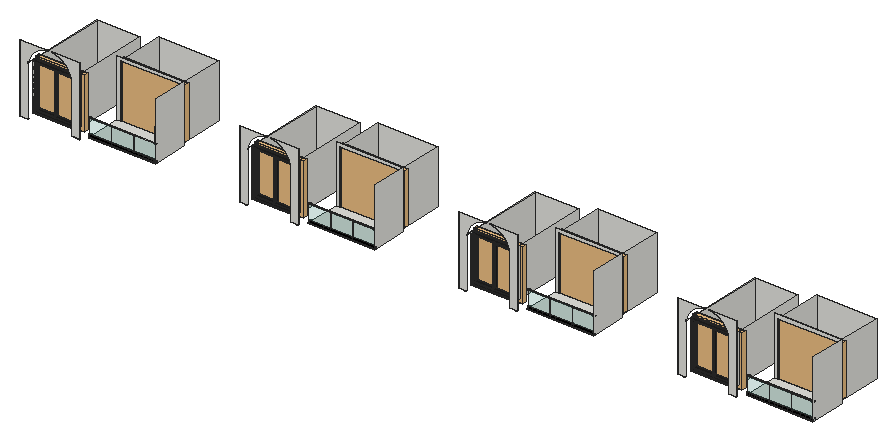
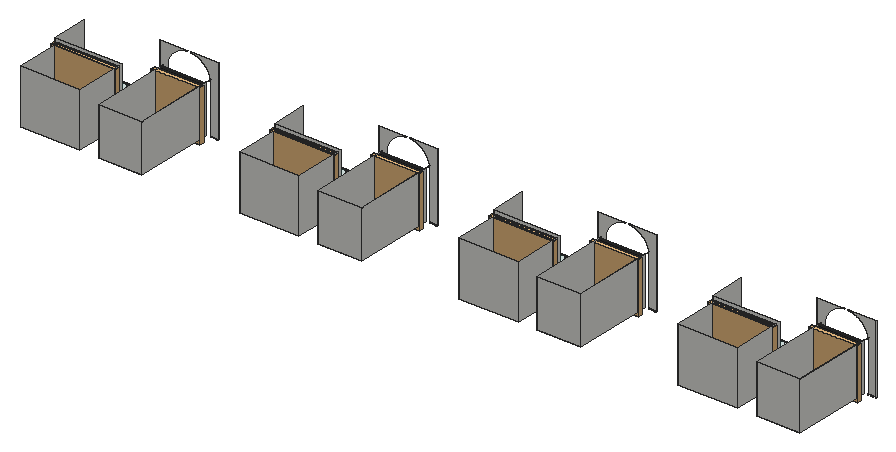
# SketchUp Ruby script. Lengths in inches.
U = 1.inch
M = Sketchup.active_model
def pt(a) = Geom::Point3d.new(a.map { |v| v * U })
def face(e, loops, mat)
  f = e.add_face(loops[0].map { |a| pt(a) })
  loops[1..].each { |l| e.add_face(l.map { |a| pt(a) }).erase! }
  f.material = f.back_material = mat if mat
  f
end
# faces: each face lists its corners as indices into pts; further lists are holes
def faces(e, pts, list, mat = nil) = list.each { |f| face(e, (f[0].is_a?(Array) ? f : [f]).map { |l| l.map { |i| pts[i] } }, mat) }
# xy, xz, yz: faces in a plane at the given z, y or x. An outline is a flat list of corners, or four numbers for a rectangle; further outlines are holes
def ring(l) = l.size == 4 ? [[l[0], l[1]], [l[2], l[1]], [l[2], l[3]], [l[0], l[3]]] : l.each_slice(2).to_a
def flat(e, list, mat, &to3) = list.each { |f| face(e, (f[0].is_a?(Array) ? f : [f]).map { |l| ring(l).map { |u, v| to3.(u, v) } }, mat) }
def xy(e, z, list, mat = nil) = flat(e, list, mat) { |x, y| [x, y, z] }
def xz(e, y, list, mat = nil) = flat(e, list, mat) { |x, z| [x, y, z] }
def yz(e, x, list, mat = nil) = flat(e, list, mat) { |y, z| [x, y, z] }
def lines(e, pts, list) = list.each { |a, b| e.add_line(pt(pts[a]), pt(pts[b])) }
# prism: a flat outline (further loops are holes) pulled along v
def prism(e, loops, v, mat = nil)
  f = face(e, loops, mat); d = Geom::Vector3d.new(v.map { |x| x * U })
  f.pushpull(f.normal.samedirection?(d) ? d.length : -d.length)
end
def box(e, o, s, mat = nil) = prism(e, [[o, [o[0] + s[0], o[1], o[2]], [o[0] + s[0], o[1] + s[1], o[2]], [o[0], o[1] + s[1], o[2]]]], [0, 0, s[2]], mat)
def at(x, y, z, deg = 0) = Geom::Transformation.translation(pt([x, y, z])) * Geom::Transformation.rotation(ORIGIN, Z_AXIS, deg.degrees)
def axes(o, x, y, z) = Geom::Transformation.new([*x, 0, *y, 0, *z, 0, *pt(o).to_a, 1])
def part(name) = M.definitions.add(name)
# library, detail: a bought-in or finely detailed component or shape, given as its bounding box
def library(name, o, s) = part(name).tap { |d| box(d.entities, o, s) }
def detail(e, o, s) = box(e.add_group.entities, o, s)
def put(e, d, t, mat = nil) = e.add_instance(d, t).tap { |i| i.material = mat if mat }
def group(e, t, mat = nil) = e.add_group.tap { |g| g.transformation = t; g.material = mat if mat }.entities
root = M.entities
M.materials.add("Glass Railing Color").color = [198, 198, 198]
M.materials.add("POT_TEXTURE_1").color = [172, 172, 172]
M.materials.add("Railing Glass").color = [63, 150, 137]
M.materials["Railing Glass"].alpha = 0.13
M.materials.add("[Color M09]").color = [0, 0, 0]
M.materials.add("[Color_009]").color = [33, 33, 33]
M.materials.add("[Color_A01]").color = [253, 112, 112]
M.materials["[Color_A01]"].alpha = 0
M.materials.add("soil1").color = [68, 55, 47]
c1 = library("Window_Curtains2",[0,-81.89,0],[92,82.37,8.12])
c2 = part("Group\#33")
prism(c2.entities,[[[22.64,0,0],[0,0,0],[0,43.31,0],[22.64,43.31,0]],[[20.67,41.34,0],[1.97,41.34,0],[1.97,1.97,0],[20.67,1.97,0]]],[0,0,1.38])
c3 = part("Group\#34")
box(c3.entities,[0,0,0],[18.7,39.37,0.39])
c4 = part("2slidwin w fix bottom")
put(c4.entities,c2,axes([1.97,0,22.15],[1,0,0],[0,0,1.25],[0,-1,0]),"[Color_009]")
put(c4.entities,c3,axes([3.9375,-0.2,24.61],[1,0,0],[0,0,1.25],[0,-1,0]),"[Color_A01]")
g1 = group(c4.entities,at(0,-0.2,0),"[Color_009]")
prism(g1,[[[47.24,0,19.69],[0,0,19.69],[0,0,78.74],[47.24,0,78.74]],[[45.28,0,22.15],[45.28,0,76.28],[1.97,0,76.28],[1.97,0,22.15]]],[0,-3.15,0])
put(c4.entities,c2,axes([22.64,-1.38,22.15],[1,0,0],[0,0,1.25],[0,-1,0]),"[Color_009]")
put(c4.entities,c3,axes([24.61,-1.57,24.61],[1,0,0],[0,0,1.25],[0,-1,0]),"[Color_A01]")
c5 = library("Sliding windows",[337.77,-0.89,0.35],[154.53,8.85,122.84])
c6 = part("Glass Rail Spacer")
box(c6.entities,[-0.5,-0.25,0],[1,0.5,1],"Glass Railing Color")
c7 = part("Group9\#1")
prism(c7.entities,[[[0.54,0,1.27],[0.38,0,1.39],[0.21,0,1.47],[0.01,0,1.5],[-0.18,0,1.48],[-0.37,0,1.41],[-0.52,0,1.29],[-0.64,0,1.13],[-0.72,0,0.96],[-0.75,0,0.76],[-0.73,0,0.57],[-0.66,0,0.38],[-0.54,0,0.23],[-0.38,0,0.11],[-0.21,0,0.03],[-0.01,0,0],[0.18,0,0.02],[0.37,0,0.09],[0.52,0,0.21],[0.64,0,0.37],[0.72,0,0.54],[0.75,0,0.74],[0.73,0,0.93],[0.66,0,1.12]]],[0,136,0],"[Color M09]")
c8 = part("Group12\#1")
xy(c8.entities,0,[[-0.5,0,0.5,136]],"Glass Railing Color")
xy(c8.entities,4,[[-0.25,0,0.25,136]],"Glass Railing Color")
xy(c8.entities,5,[[-0.5,0,-0.25,136],[0.25,0,0.5,136]],"[Color M09]")
xz(c8.entities,0,[[-0.5,0,0.5,0,0.5,5,0.25,5,0.25,4,-0.25,4,-0.25,5,-0.5,5]],"Glass Railing Color")
xz(c8.entities,136,[[-0.5,0,-0.5,5,-0.25,5,-0.25,4,0.25,4,0.25,5,0.5,5,0.5,0]],"Glass Railing Color")
yz(c8.entities,-0.5,[[0,0,136,5]],"[Color M09]")
yz(c8.entities,-0.25,[[0,4,136,5]],"[Color M09]")
yz(c8.entities,0.25,[[0,4,136,5]],"[Color M09]")
yz(c8.entities,0.5,[[0,0,136,5]],"[Color M09]")
c9 = part("Group13\#1")
box(c9.entities,[-0.1875,0,0],[0.375,44,30],"Railing Glass")
c10 = part("Group14\#1")
box(c10.entities,[-0.1875,0,0],[0.375,44,30],"Railing Glass")
c11 = part("Group15\#1")
box(c11.entities,[-0.1875,0,0],[0.375,44,30],"Railing Glass")
c12 = part("Glass Railing")
put(c12.entities,c6,at(0,0,4))
put(c12.entities,c6,at(45,0,4))
put(c12.entities,c6,at(90,0,4))
put(c12.entities,c6,at(135,0,4))
put(c12.entities,c7,at(-0.5,0,34,-90),"Glass Railing Color")
put(c12.entities,c8,at(-0.5,0,0,-90),"Glass Railing Color")
put(c12.entities,c9,at(0.5,0,4,-90),"Railing Glass")
put(c12.entities,c10,at(45.5,0,4,-90),"Railing Glass")
put(c12.entities,c11,at(90.5,0,4,-90),"Railing Glass")
c13 = library("Group\#96",[-662.41,217.3,320.04],[397.32,658.3,1732.06])
c14 = library("Group\#98",[-299.2,181.55,262.58],[360.65,735.71,1258.34])
c15 = library("Group\#93",[-1038.76,656.55,345.34],[733.18,460.51,2065.7])
c16 = library("Group\#91",[-445.29,890.31,329.28],[284.3,304.08,2023.29])
c17 = library("Group\#94",[-733.48,439.625,202.64],[456.28,533.12,1536.78])
c18 = library("Group\#97",[-455.56,899.32,410.78],[341.21,610.33,1581.5])
c19 = library("Group\#90",[-516.34,626.77,-4.5625],[517.73,515.95,418.98])
c20 = library("Group\#95",[-249.24,914.85,310.18],[345.55,647.95,1307.93])
c21 = library("Group\#92",[-277.97,488.68,287.26],[362.84,405.94,1768.54])
c22 = library("Group\#89",[-468.76,669.89,380.1875],[424.36,427.47,41.99])
c23 = part("Potted broadleaf plant")
put(c23.entities,c13,at(1038.76,-181.55,4.5625))
put(c23.entities,c14,at(1038.76,-181.55,4.5625))
put(c23.entities,c15,at(1038.76,-181.55,4.5625))
put(c23.entities,c16,at(1038.76,-181.55,4.5625))
put(c23.entities,c17,at(1038.76,-181.55,4.5625))
put(c23.entities,c18,at(1038.76,-181.55,4.5625))
put(c23.entities,c19,at(1038.76,-181.55,4.5625),"POT_TEXTURE_1")
put(c23.entities,c20,at(1038.76,-181.55,4.5625))
put(c23.entities,c21,at(1038.76,-181.55,4.5625))
put(c23.entities,c22,at(1038.76,-181.55,4.5625),"soil1")
xy(root,132.03,[[159.1,224.6875,175,225.16],[263,224.6875,278.75,225.16],[603.1,224.6875,619,225.16],[707,224.6875,722.75,225.16],[1047.1,224.6875,1063,225.16],
  [1151,224.6875,1166.75,225.16],[1491.1,224.6875,1507,225.16],[1595,224.6875,1610.75,225.16]])
xy(root,132.5,[[159.1,224.6875,175,225.16],[263,224.6875,278.75,225.16],[603.1,224.6875,619,225.16],[707,224.6875,722.75,225.16],[1047.1,224.6875,1063,225.16],
  [1151,224.6875,1166.75,225.16],[1491.1,224.6875,1507,225.16],[1595,224.6875,1610.75,225.16]])
xy(root,139,[[294,229.25,429,229.25,429,301.25,422,301.25,422,398.125,301,398.125,301,301.25,294,301.25],[738,229.25,873,229.25,873,301.25,866,301.25,866,398.125,745,398.125,745,301.25,738,301.25],[1182,229.25,1317,229.25,1317,301.25,1310,301.25,1310,398.125,1189,398.125,1189,301.25,1182,301.25],[1626,229.25,1761,229.25,1761,301.25,1754,301.25,1754,398.125,1633,398.125,1633,301.25,1626,301.25],[175,236.25,263,398.125],
  [619,236.25,707,398.125],[1063,236.25,1151,398.125],[1507,236.25,1595,398.125]])
xz(root,224.6875,[[159.1,132.5,175,132.5,175,235.48,175.125,235.48,175.26,236.08,175.4,236.68,175.55,237.28,175.7,237.875,175.87,238.47,176.04,239.06,176.22,239.65,176.41,240.24,176.61,240.82,177.03,241.98,177.25,242.56,177.48,243.13,177.72,243.7,177.97,244.26,178.22,244.83,178.48,245.38,178.75,245.94,179.02,246.49,179.31,247.04,179.6,247.58,180.2,248.66,180.84,249.72,181.16,250.24,181.5,250.76,181.84,251.27,182.19,251.78,182.91,252.78,183.65,253.76,184.04,254.25,184.43,254.72,184.82,255.2,185.23,255.66,185.64,256.125,186.05,256.58,186.47,257.03,186.9,257.48,187.77,258.35,188.67,259.19,189.13,259.61,189.59,260.02,190.06,260.42,190.53,260.8125,191.01,261.2,191.99,261.96,192.48,262.32,192.98,262.68,193.49,263.04,194,263.39,194.51,263.73,195.55,264.39,196.08,264.7,196.61,265.02,197.69,265.62,198.24,265.91,198.79,266.1875,199.34,266.46,199.89,266.73,200.45,266.99,201.02,267.24,201.58,267.48,202.15,267.72,202.73,267.94,203.3,268.16,203.88,268.375,204.46,268.58,205.05,268.78,206.23,269.14,207.41,269.48,208.61,269.78,209.21,269.92,209.8125,270.05,210.42,270.17,211.02,270.29,212.24,270.49,212.85,270.58,213.46,270.66,214.08,270.73,214.6875,270.79,215.3,270.85,215.92,270.89,159.1,270.89],[263,132.5,278.75,132.5,278.75,270.89,222.08,270.89,222.66,270.85,223.27,270.8,225.1,270.59,225.7,270.5,226.3,270.4,226.91,270.3,227.51,270.1875,228.11,270.07,228.71,269.94,229.3,269.81,229.9,269.66,230.49,269.51,231.08,269.35,231.67,269.18,232.25,269,232.84,268.82,233.42,268.63,233.99,268.43,234.57,268.22,235.14,268.01,236.28,267.55,236.84,267.3125,237.4,267.07,237.96,266.8125,238.51,266.55,239.06,266.28,239.6,266.01,240.15,265.72,240.68,265.43,241.22,265.14,241.75,264.83,242.27,264.52,242.79,264.2,243.31,263.87,243.82,263.54,244.33,263.2,244.83,262.85,245.33,262.49,245.82,262.13,246.3125,261.77,246.8,261.39,247.28,261.01,247.75,260.625,248.22,260.23,248.68,259.83,249.14,259.42,249.59,259.01,250.47,258.17,250.91,257.74,251.34,257.3,251.76,256.86,252.58,255.96,252.99,255.5,253.39,255.03,253.78,254.5625,254.16,254.09,254.54,253.61,254.91,253.125,255.28,252.63,255.64,252.14,255.99,251.64,256.33,251.13,256.67,250.625,257,250.11,257.33,249.59,257.64,249.07,258.26,248.01,258.55,247.48,258.84,246.9375,259.12,246.39,259.39,245.85,259.66,245.3,259.92,244.74,260.17,244.18,260.65,243.06,261.1,241.92,261.31,241.35,261.71,240.19,261.9,239.61,262.08,239.03,262.42,237.85,262.58,237.26,262.73,236.67,262.87,236.07,263,235.48],[603.1,132.5,619,132.5,619,235.48,619.125,235.48,619.26,236.08,619.4,236.68,619.55,237.28,619.7,237.875,619.87,238.47,620.04,239.06,620.22,239.65,620.41,240.24,620.61,240.82,621.03,241.98,621.25,242.56,621.48,243.13,621.72,243.7,621.97,244.26,622.22,244.83,622.48,245.38,622.75,245.94,623.02,246.49,623.31,247.04,623.6,247.58,624.2,248.66,624.84,249.72,625.16,250.24,625.5,250.76,625.84,251.27,626.19,251.78,626.91,252.78,627.65,253.76,628.04,254.25,628.43,254.72,628.82,255.2,629.23,255.66,629.64,256.125,630.05,256.58,630.47,257.03,630.9,257.48,631.77,258.35,632.67,259.19,633.13,259.61,633.59,260.02,634.06,260.42,634.53,260.8125,635.01,261.2,635.99,261.96,636.48,262.32,636.98,262.68,637.49,263.04,638,263.39,638.51,263.73,639.55,264.39,640.08,264.7,640.61,265.02,641.69,265.62,642.24,265.91,642.79,266.1875,643.34,266.46,643.89,266.73,644.45,266.99,645.02,267.24,645.58,267.48,646.15,267.72,646.73,267.94,647.3,268.16,647.88,268.375,648.46,268.58,649.05,268.78,650.23,269.14,651.41,269.48,652.61,269.78,653.21,269.92,653.8125,270.05,654.42,270.17,655.02,270.29,656.24,270.49,656.85,270.58,657.46,270.66,658.08,270.73,658.6875,270.79,659.3,270.85,659.92,270.89,603.1,270.89],[707,132.5,722.75,132.5,722.75,270.89,666.08,270.89,666.66,270.85,667.27,270.8,669.1,270.59,669.7,270.5,670.3,270.4,670.91,270.3,671.51,270.1875,672.11,270.07,672.71,269.94,673.3,269.81,673.9,269.66,674.49,269.51,675.08,269.35,675.67,269.18,676.25,269,676.84,268.82,677.42,268.63,677.99,268.43,678.57,268.22,679.14,268.01,680.28,267.55,680.84,267.3125,681.4,267.07,681.96,266.8125,682.51,266.55,683.06,266.28,683.6,266.01,684.15,265.72,684.68,265.43,685.22,265.14,685.75,264.83,686.27,264.52,686.79,264.2,687.31,263.87,687.82,263.54,688.33,263.2,688.83,262.85,689.33,262.49,689.82,262.13,690.3125,261.77,690.8,261.39,691.28,261.01,691.75,260.625,692.22,260.23,692.68,259.83,693.14,259.42,693.59,259.01,694.47,258.17,694.91,257.74,695.34,257.3,695.76,256.86,696.58,255.96,696.99,255.5,697.39,255.03,697.78,254.5625,698.16,254.09,698.54,253.61,698.91,253.125,699.28,252.63,699.64,252.14,699.99,251.64,700.33,251.13,700.67,250.625,701,250.11,701.33,249.59,701.64,249.07,702.26,248.01,702.55,247.48,702.84,246.9375,703.12,246.39,703.39,245.85,703.66,245.3,703.92,244.74,704.17,244.18,704.65,243.06,705.1,241.92,705.31,241.35,705.71,240.19,705.9,239.61,706.08,239.03,706.42,237.85,706.58,237.26,706.73,236.67,706.87,236.07,707,235.48],[1047.1,132.5,1063,132.5,1063,235.48,1063.125,235.48,1063.26,236.08,1063.4,236.68,1063.55,237.28,1063.7,237.875,1063.87,238.47,1064.04,239.06,1064.22,239.65,1064.41,240.24,1064.61,240.82,1065.03,241.98,1065.25,242.56,1065.48,243.13,1065.72,243.7,1065.97,244.26,1066.22,244.83,1066.48,245.38,1066.75,245.94,1067.02,246.49,1067.31,247.04,1067.6,247.58,1068.2,248.66,1068.84,249.72,1069.16,250.24,1069.5,250.76,1069.84,251.27,1070.19,251.78,1070.91,252.78,1071.65,253.76,1072.04,254.25,1072.43,254.72,1072.82,255.2,1073.23,255.66,1073.64,256.125,1074.05,256.58,1074.47,257.03,1074.9,257.48,1075.77,258.35,1076.67,259.19,1077.13,259.61,1077.59,260.02,1078.06,260.42,1078.53,260.8125,1079.01,261.2,1079.99,261.96,1080.48,262.32,1080.98,262.68,1081.49,263.04,1082,263.39,1082.51,263.73,1083.55,264.39,1084.08,264.7,1084.61,265.02,1085.69,265.62,1086.24,265.91,1086.79,266.1875,1087.34,266.46,1087.89,266.73,1088.45,266.99,1089.02,267.24,1089.58,267.48,1090.15,267.72,1090.73,267.94,1091.3,268.16,1091.88,268.375,1092.46,268.58,1093.05,268.78,1094.23,269.14,1095.41,269.48,1096.61,269.78,1097.21,269.92,1097.8125,270.05,1098.42,270.17,1099.02,270.29,1100.24,270.49,1100.85,270.58,1101.46,270.66,1102.08,270.73,1102.6875,270.79,1103.3,270.85,1103.92,270.89,1047.1,270.89],
  [1151,132.5,1166.75,132.5,1166.75,270.89,1110.08,270.89,1110.66,270.85,1111.27,270.8,1113.1,270.59,1113.7,270.5,1114.3,270.4,1114.91,270.3,1115.51,270.1875,1116.11,270.07,1116.71,269.94,1117.3,269.81,1117.9,269.66,1118.49,269.51,1119.08,269.35,1119.67,269.18,1120.25,269,1120.84,268.82,1121.42,268.63,1121.99,268.43,1122.57,268.22,1123.14,268.01,1124.28,267.55,1124.84,267.3125,1125.4,267.07,1125.96,266.8125,1126.51,266.55,1127.06,266.28,1127.6,266.01,1128.15,265.72,1128.68,265.43,1129.22,265.14,1129.75,264.83,1130.27,264.52,1130.79,264.2,1131.31,263.87,1131.82,263.54,1132.33,263.2,1132.83,262.85,1133.33,262.49,1133.82,262.13,1134.3125,261.77,1134.8,261.39,1135.28,261.01,1135.75,260.625,1136.22,260.23,1136.68,259.83,1137.14,259.42,1137.59,259.01,1138.47,258.17,1138.91,257.74,1139.34,257.3,1139.76,256.86,1140.58,255.96,1140.99,255.5,1141.39,255.03,1141.78,254.5625,1142.16,254.09,1142.54,253.61,1142.91,253.125,1143.28,252.63,1143.64,252.14,1143.99,251.64,1144.33,251.13,1144.67,250.625,1145,250.11,1145.33,249.59,1145.64,249.07,1146.26,248.01,1146.55,247.48,1146.84,246.9375,1147.12,246.39,1147.39,245.85,1147.66,245.3,1147.92,244.74,1148.17,244.18,1148.65,243.06,1149.1,241.92,1149.31,241.35,1149.71,240.19,1149.9,239.61,1150.08,239.03,1150.42,237.85,1150.58,237.26,1150.73,236.67,1150.87,236.07,1151,235.48],[1491.1,132.5,1507,132.5,1507,235.48,1507.125,235.48,1507.26,236.08,1507.4,236.68,1507.55,237.28,1507.7,237.875,1507.87,238.47,1508.04,239.06,1508.22,239.65,1508.41,240.24,1508.61,240.82,1509.03,241.98,1509.25,242.56,1509.48,243.13,1509.72,243.7,1509.97,244.26,1510.22,244.83,1510.48,245.38,1510.75,245.94,1511.02,246.49,1511.31,247.04,1511.6,247.58,1512.2,248.66,1512.84,249.72,1513.16,250.24,1513.5,250.76,1513.84,251.27,1514.19,251.78,1514.91,252.78,1515.65,253.76,1516.04,254.25,1516.43,254.72,1516.82,255.2,1517.23,255.66,1517.64,256.125,1518.05,256.58,1518.47,257.03,1518.9,257.48,1519.77,258.35,1520.67,259.19,1521.13,259.61,1521.59,260.02,1522.06,260.42,1522.53,260.8125,1523.01,261.2,1523.99,261.96,1524.48,262.32,1524.98,262.68,1525.49,263.04,1526,263.39,1526.51,263.73,1527.55,264.39,1528.08,264.7,1528.61,265.02,1529.69,265.62,1530.24,265.91,1530.79,266.1875,1531.34,266.46,1531.89,266.73,1532.45,266.99,1533.02,267.24,1533.58,267.48,1534.15,267.72,1534.73,267.94,1535.3,268.16,1535.88,268.375,1536.46,268.58,1537.05,268.78,1538.23,269.14,1539.41,269.48,1540.61,269.78,1541.21,269.92,1541.8125,270.05,1542.42,270.17,1543.02,270.29,1544.24,270.49,1544.85,270.58,1545.46,270.66,1546.08,270.73,1546.6875,270.79,1547.3,270.85,1547.92,270.89,1491.1,270.89],[1595,132.5,1610.75,132.5,1610.75,270.89,1554.08,270.89,1554.66,270.85,1555.27,270.8,1557.1,270.59,1557.7,270.5,1558.3,270.4,1558.91,270.3,1559.51,270.1875,1560.11,270.07,1560.71,269.94,1561.3,269.81,1561.9,269.66,1562.49,269.51,1563.08,269.35,1563.67,269.18,1564.25,269,1564.84,268.82,1565.42,268.63,1565.99,268.43,1566.57,268.22,1567.14,268.01,1568.28,267.55,1568.84,267.3125,1569.4,267.07,1569.96,266.8125,1570.51,266.55,1571.06,266.28,1571.6,266.01,1572.15,265.72,1572.68,265.43,1573.22,265.14,1573.75,264.83,1574.27,264.52,1574.79,264.2,1575.31,263.87,1575.82,263.54,1576.33,263.2,1576.83,262.85,1577.33,262.49,1577.82,262.13,1578.3125,261.77,1578.8,261.39,1579.28,261.01,1579.75,260.625,1580.22,260.23,1580.68,259.83,1581.14,259.42,1581.59,259.01,1582.47,258.17,1582.91,257.74,1583.34,257.3,1583.76,256.86,1584.58,255.96,1584.99,255.5,1585.39,255.03,1585.78,254.5625,1586.16,254.09,1586.54,253.61,1586.91,253.125,1587.28,252.63,1587.64,252.14,1587.99,251.64,1588.33,251.13,1588.67,250.625,1589,250.11,1589.33,249.59,1589.64,249.07,1590.26,248.01,1590.55,247.48,1590.84,246.9375,1591.12,246.39,1591.39,245.85,1591.66,245.3,1591.92,244.74,1592.17,244.18,1592.65,243.06,1593.1,241.92,1593.31,241.35,1593.71,240.19,1593.9,239.61,1594.08,239.03,1594.42,237.85,1594.58,237.26,1594.73,236.67,1594.87,236.07,1595,235.48]])
xz(root,229.25,[[175,234.87,175.125,235.48,175,235.48],[619,234.87,619.125,235.48,619,235.48],[1063,234.87,1063.125,235.48,1063,235.48],[1507,234.87,1507.125,235.48,1507,235.48]])
xz(root,301.25,[[294,139,301,139,301,249,422,249,422,139,429,139,429,256,294,256],[738,139,745,139,745,249,866,249,866,139,873,139,873,256,738,256],[1182,139,1189,139,1189,249,1310,249,1310,139,1317,139,1317,256,1182,256],[1626,139,1633,139,1633,249,1754,249,1754,139,1761,139,1761,256,1626,256]])
xz(root,398.125,[[175,139,263,139,263,235.48,175.125,235.48,175,234.87],[301,139,422,249],[619,139,707,139,707,235.48,619.125,235.48,619,234.87],[745,139,866,249],[1063,139,1151,139,1151,235.48,1063.125,235.48,1063,234.87],
  [1189,139,1310,249],[1507,139,1595,139,1595,235.48,1507.125,235.48,1507,234.87],[1633,139,1754,249]])
yz(root,159.1,[[224.6875,132.5,225.16,270.89]])
yz(root,175,[[236.25,139,398.125,234.87],[224.6875,234.87,229.25,235.48]])
yz(root,263,[[236.25,139,398.125,235.48]])
yz(root,278.75,[[224.6875,132.5,225.16,270.89]])
yz(root,301,[[301.25,139,398.125,249]])
yz(root,422,[[301.25,139,398.125,249]])
yz(root,429,[[229.25,139,301.25,256]])
yz(root,603.1,[[224.6875,132.5,225.16,270.89]])
yz(root,619,[[236.25,139,398.125,234.87],[224.6875,234.87,229.25,235.48]])
yz(root,707,[[236.25,139,398.125,235.48]])
yz(root,722.75,[[224.6875,132.5,225.16,270.89]])
yz(root,745,[[301.25,139,398.125,249]])
yz(root,866,[[301.25,139,398.125,249]])
yz(root,873,[[229.25,139,301.25,256]])
yz(root,1047.1,[[224.6875,132.5,225.16,270.89]])
yz(root,1063,[[236.25,139,398.125,234.87],[224.6875,234.87,229.25,235.48]])
yz(root,1151,[[236.25,139,398.125,235.48]])
yz(root,1166.75,[[224.6875,132.5,225.16,270.89]])
yz(root,1189,[[301.25,139,398.125,249]])
yz(root,1310,[[301.25,139,398.125,249]])
yz(root,1317,[[229.25,139,301.25,256]])
yz(root,1491.1,[[224.6875,132.5,225.16,270.89]])
yz(root,1507,[[236.25,139,398.125,234.87],[224.6875,234.87,229.25,235.48]])
yz(root,1595,[[236.25,139,398.125,235.48]])
yz(root,1610.75,[[224.6875,132.5,225.16,270.89]])
yz(root,1633,[[301.25,139,398.125,249]])
yz(root,1754,[[301.25,139,398.125,249]])
yz(root,1761,[[229.25,139,301.25,256]])
p = [[175.125,229.25,235.48],[175,229.25,234.87],[175,236.25,234.87],[175,398.125,234.87],[175.125,398.125,235.48],[175.125,236.25,235.48],
  [619.125,229.25,235.48],[619,229.25,234.87],[619,236.25,234.87],[619,398.125,234.87],[619.125,398.125,235.48],[619.125,236.25,235.48],
  [1063.125,229.25,235.48],[1063,229.25,234.87],[1063,236.25,234.87],[1063,398.125,234.87],[1063.125,398.125,235.48],[1063.125,236.25,235.48],
  [1507.125,229.25,235.48],[1507,229.25,234.87],[1507,236.25,234.87],[1507,398.125,234.87],[1507.125,398.125,235.48],[1507.125,236.25,235.48]]
faces(root,p,[[0,1,2,3,4,5],[6,7,8,9,10,11],[12,13,14,15,16,17],[18,19,20,21,22,23]])
put(root,c1,axes([171.28,256.24,234.88],[1.07666,0,0],[0,0,1.25],[0,-1,0]))
put(root,c1,axes([615.28,256.24,234.88],[1.07666,0,0],[0,0,1.25],[0,-1,0]))
put(root,c1,axes([1059.28,256.24,234.88],[1.07666,0,0],[0,0,1.25],[0,-1,0]))
put(root,c1,axes([1503.28,256.24,234.88],[1.07666,0,0],[0,0,1.25],[0,-1,0]))
put(root,c4,axes([175,243.6,106.84],[1.86267,0,0],[0,1.5,0],[0,0,1.63366]))
put(root,c4,axes([619,243.6,106.84],[1.86267,0,0],[0,1.5,0],[0,0,1.63366]))
put(root,c4,axes([1063,243.6,106.84],[1.86267,0,0],[0,1.5,0],[0,0,1.63366]))
put(root,c4,axes([1507,243.6,106.84],[1.86267,0,0],[0,1.5,0],[0,0,1.63366]))
put(root,c5,axes([36.53,304.2,138.69],[0.783,0,0],[0,0.74,0],[0,0,0.89551]))
put(root,c12,at(294,231.84,139))
put(root,c5,axes([480.53,304.2,138.69],[0.783,0,0],[0,0.74,0],[0,0,0.89551]))
put(root,c12,at(738,231.84,139))
put(root,c5,axes([924.53,304.2,138.69],[0.783,0,0],[0,0.74,0],[0,0,0.89551]))
put(root,c12,at(1182,231.84,139))
put(root,c5,axes([1368.53,304.2,138.69],[0.783,0,0],[0,0.74,0],[0,0,0.89551]))
put(root,c12,at(1626,231.84,139))
put(root,c23,axes([394.35,298.61,139.25],[0,-0.0242,0],[0.0242,0,0],[0,0,0.02319]))
put(root,c23,axes([838.35,298.61,139.25],[0,-0.0242,0],[0.0242,0,0],[0,0,0.02319]))
put(root,c23,axes([1282.35,298.61,139.25],[0,-0.0242,0],[0.0242,0,0],[0,0,0.02319]))
put(root,c23,axes([1726.35,298.61,139.25],[0,-0.0242,0],[0.0242,0,0],[0,0,0.02319]))
put(root,c1,axes([297.16,312.87,248.4],[1.43304,0,0],[0,0,1.25],[0,-1,0]))
put(root,c1,axes([741.16,312.87,248.4],[1.43304,0,0],[0,0,1.25],[0,-1,0]))
put(root,c1,axes([1185.16,312.87,248.4],[1.43304,0,0],[0,0,1.25],[0,-1,0]))
put(root,c1,axes([1629.16,312.87,248.4],[1.43304,0,0],[0,0,1.25],[0,-1,0]))
